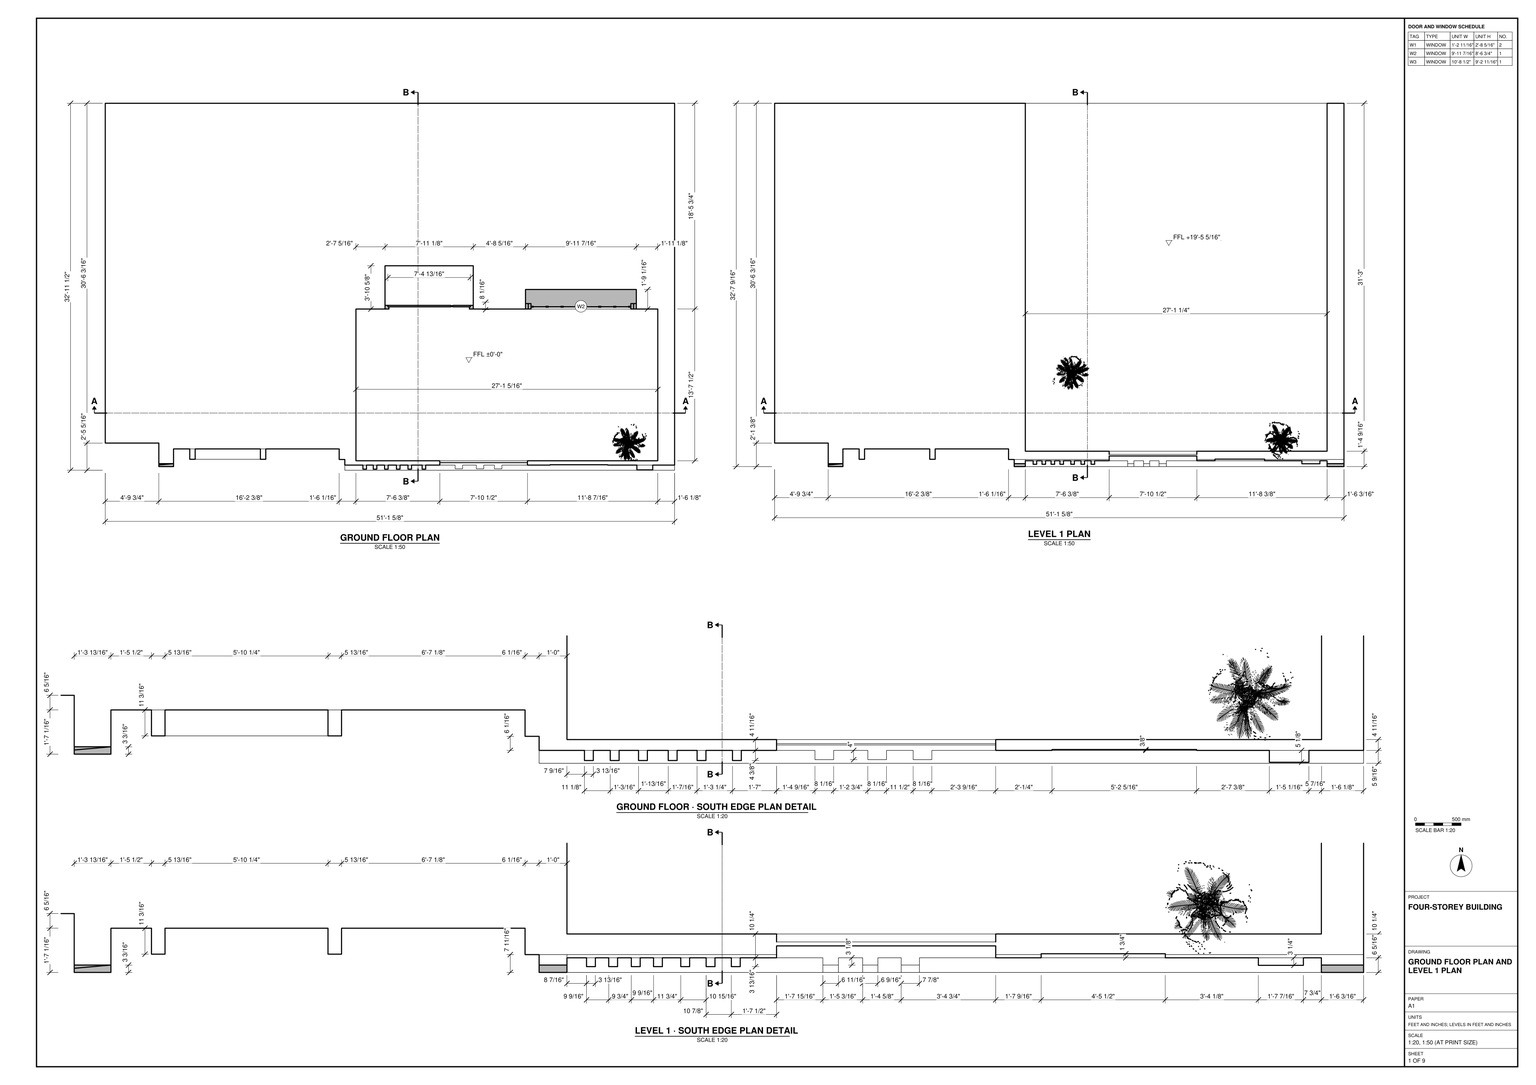
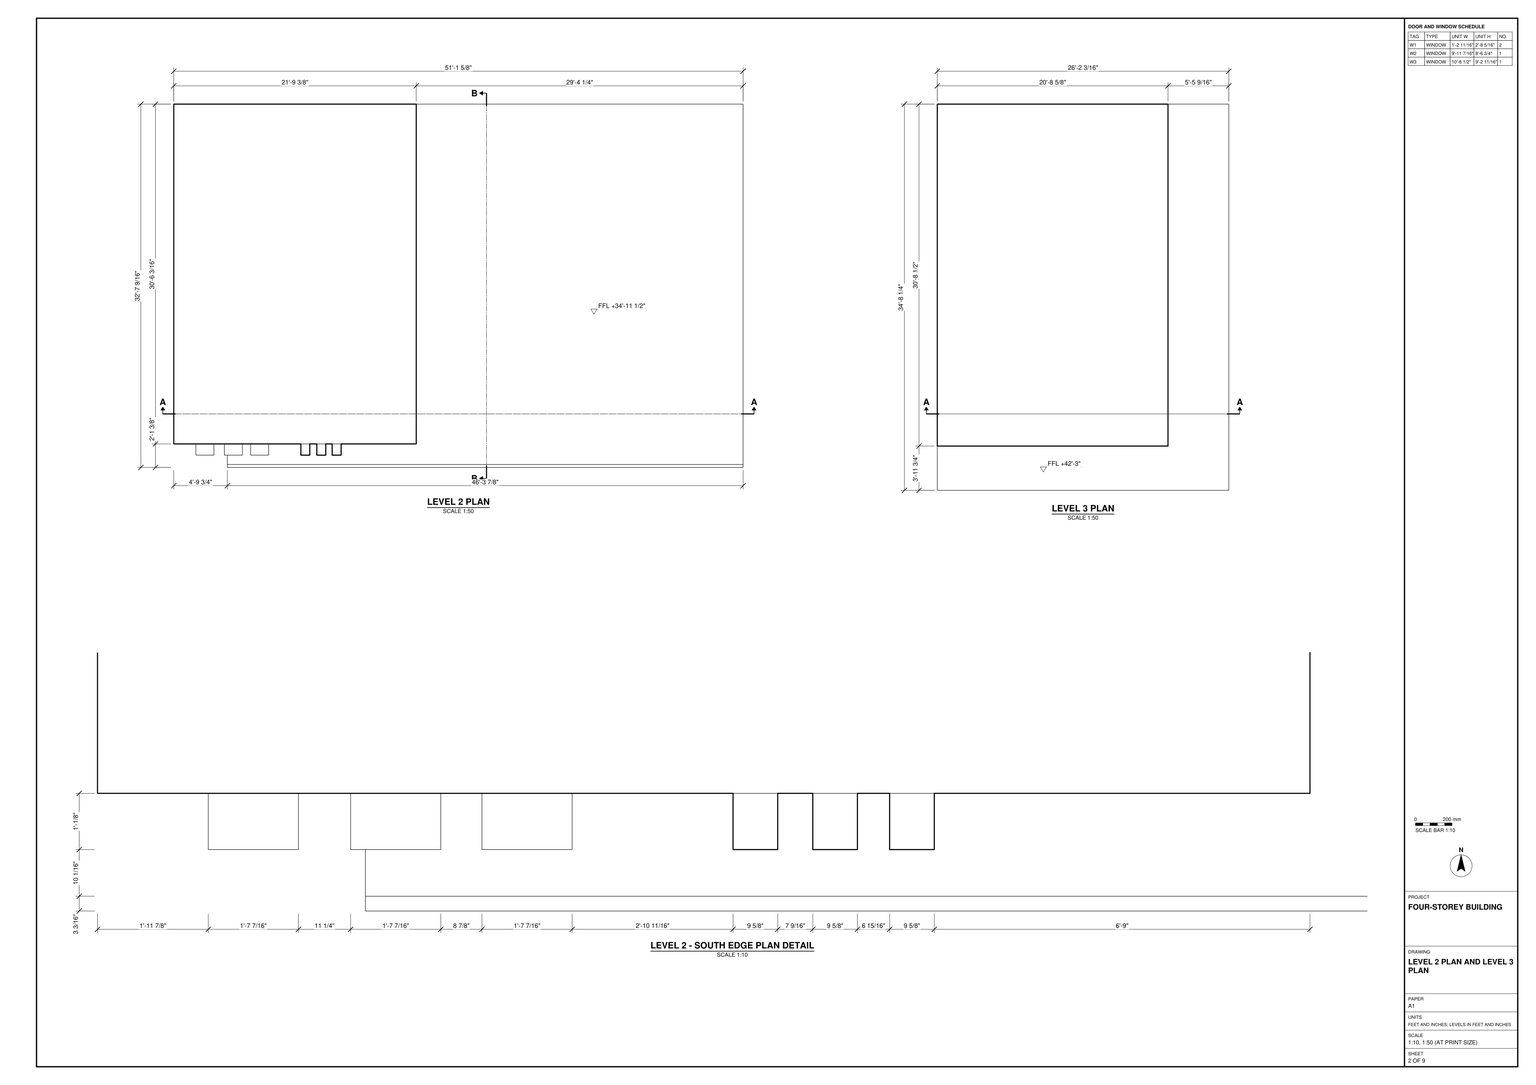
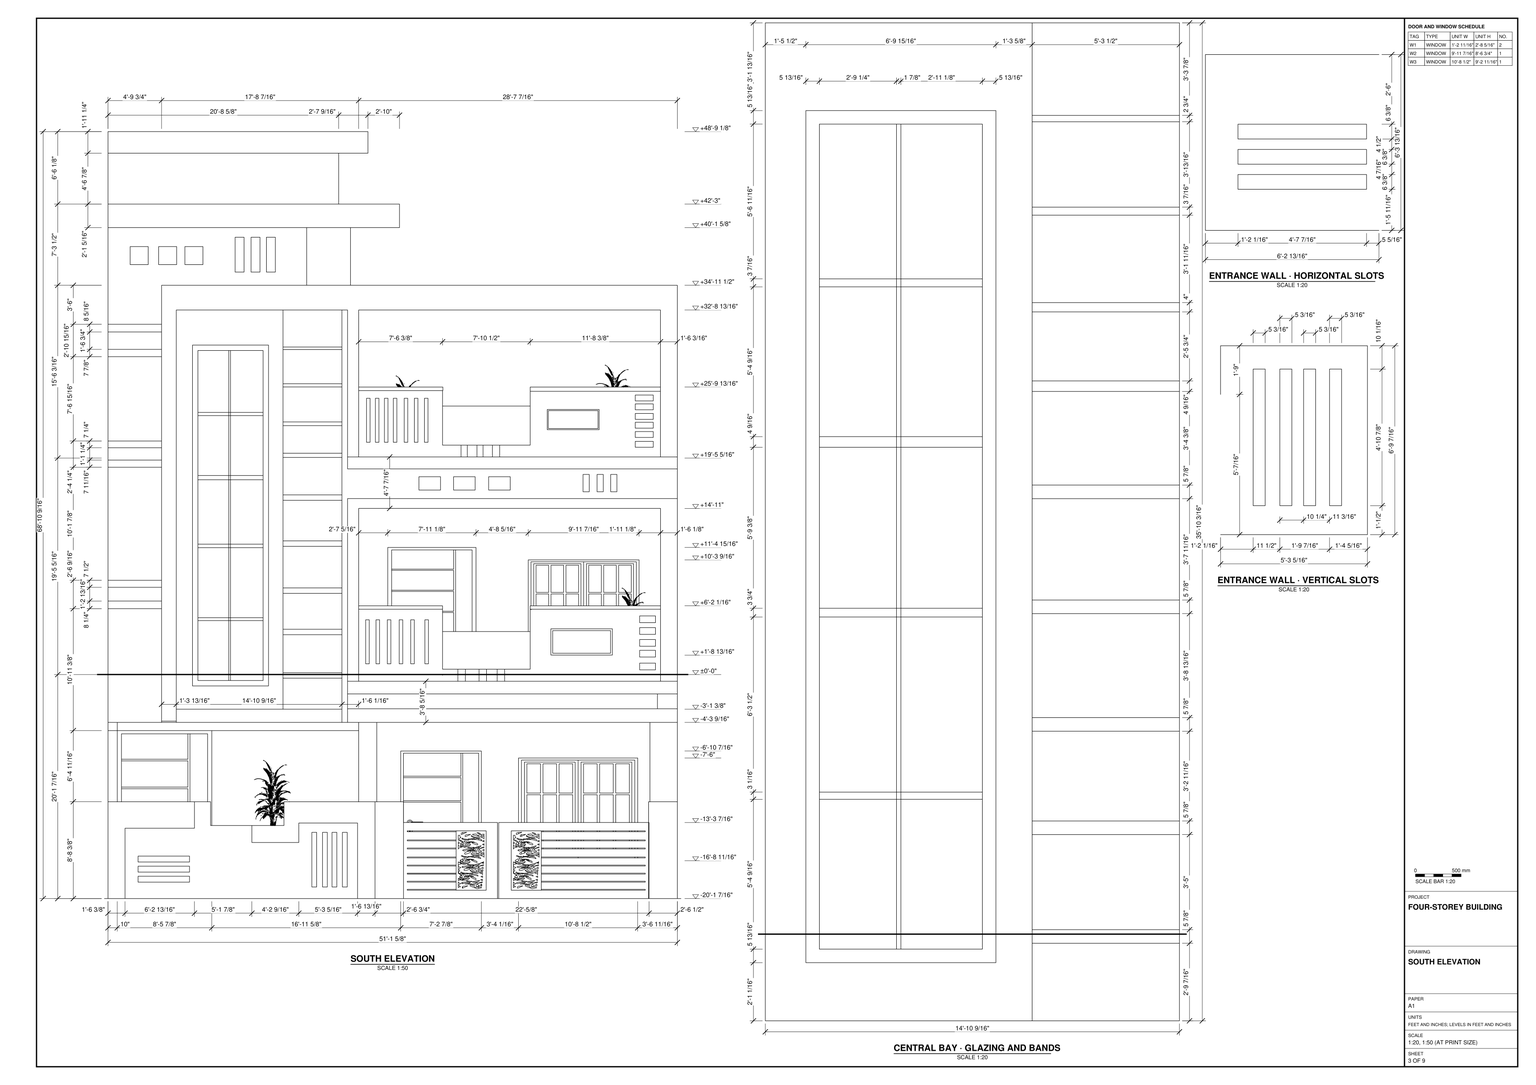
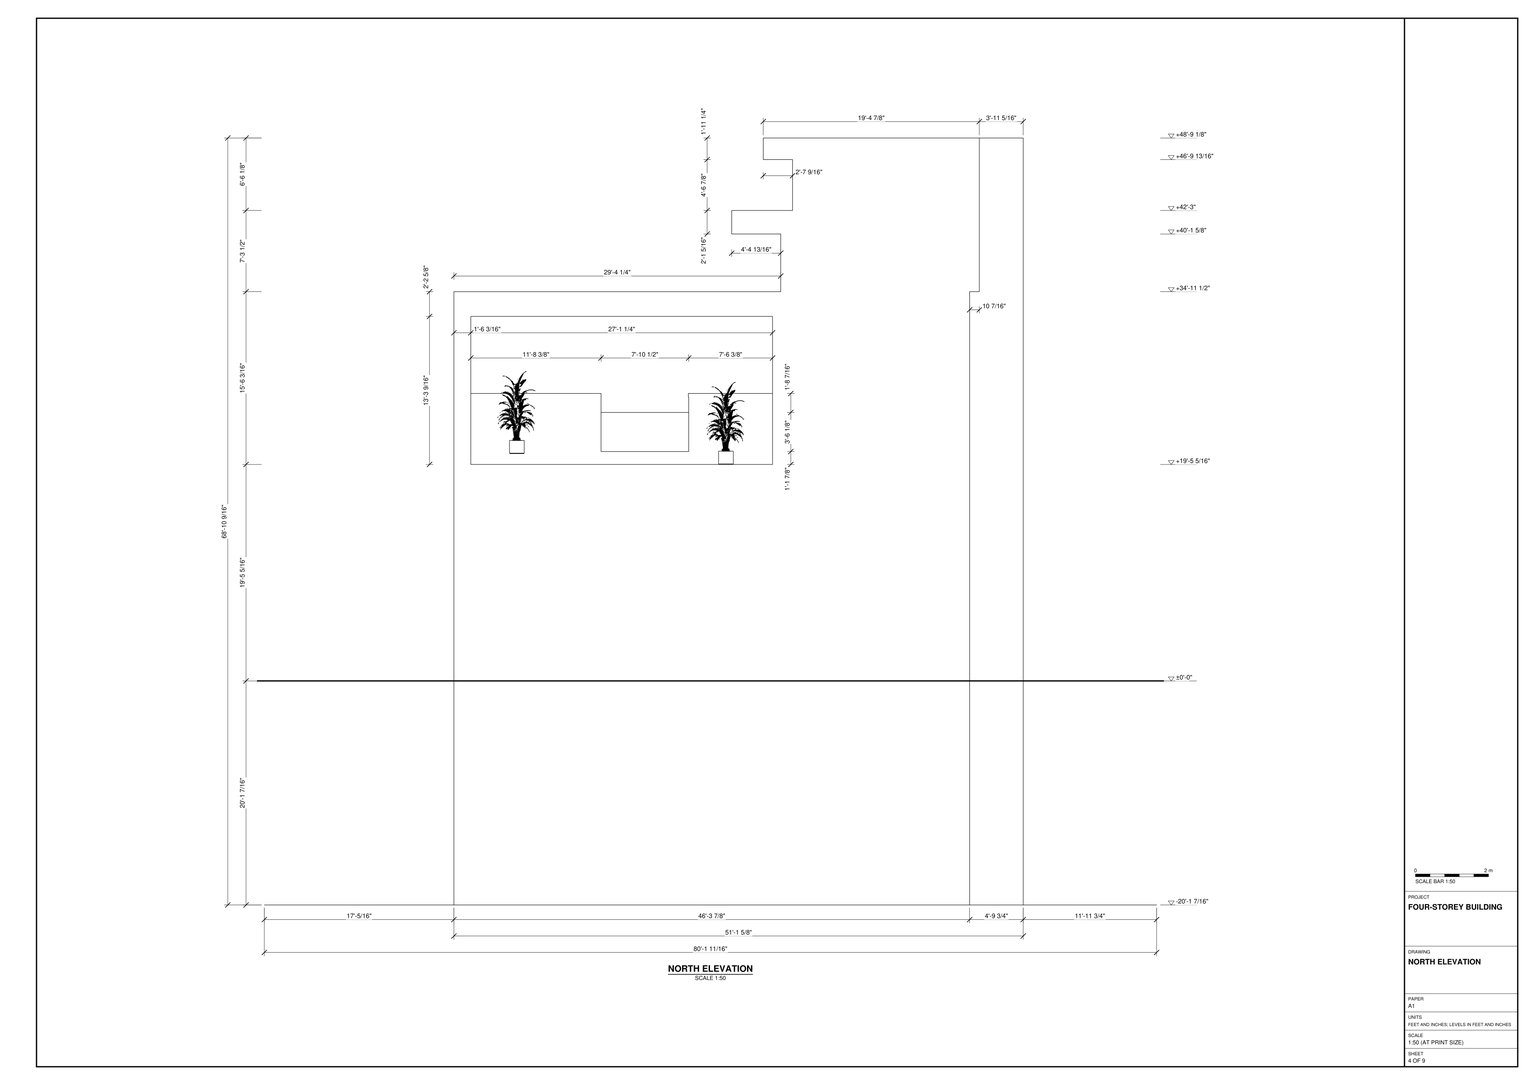
Build the four-storey building in SketchUp from task_files/diagram_01.pdf. Work in feet and inches. The complete model shall measure 80'-1 11/16" along X, 87'-11 5/8" along Y and 68'-10 9/16" along Z. Set the ground-floor datum at ±0'-0" and the successive floor levels at +19'-5 5/16", +34'-11 1/2" and +42'-3". Use the south elevation to locate the entrance frontage below the ground-floor datum.

Follow the footprint at each level rather than extruding one plan through the full height. Model the walls at their drawn thicknesses, and use the enlarged south-edge plans to shape the recesses and projections. Include the floor slabs, door and window openings, stacked balconies and the narrower upper volume with its projecting flat roof edges. On the south face, distinguish the tall divided glazing from the horizontally banded strip beside it. Reproduce the balcony parapet openings, the slotted entrance wall and the slatted gates with screen inserts. Decor and loose items, including the plants, may be any suitable library components placed where shown.

Keep walls, slabs and roof elements in separate groups or components, and do the same for each furniture or joinery piece shown. Use components for repeated parts. Save one SketchUp model as output_files/four_storey_building_and_its_south_entrance_frontage.skp.

# SketchUp Ruby script. Lengths in inches.
U = 1.inch
M = Sketchup.active_model
def pt(a) = Geom::Point3d.new(a.map { |v| v * U })
def face(e, loops, mat)
  f = e.add_face(loops[0].map { |a| pt(a) })
  loops[1..].each { |l| e.add_face(l.map { |a| pt(a) }).erase! }
  f.material = f.back_material = mat if mat
  f
end
# faces: each face lists its corners as indices into pts; further lists are holes
def faces(e, pts, list, mat = nil) = list.each { |f| face(e, (f[0].is_a?(Array) ? f : [f]).map { |l| l.map { |i| pts[i] } }, mat) }
# xy, xz, yz: faces in a plane at the given z, y or x. An outline is a flat list of corners, or four numbers for a rectangle; further outlines are holes
def ring(l) = l.size == 4 ? [[l[0], l[1]], [l[2], l[1]], [l[2], l[3]], [l[0], l[3]]] : l.each_slice(2).to_a
def flat(e, list, mat, &to3) = list.each { |f| face(e, (f[0].is_a?(Array) ? f : [f]).map { |l| ring(l).map { |u, v| to3.(u, v) } }, mat) }
def xy(e, z, list, mat = nil) = flat(e, list, mat) { |x, y| [x, y, z] }
def xz(e, y, list, mat = nil) = flat(e, list, mat) { |x, z| [x, y, z] }
def yz(e, x, list, mat = nil) = flat(e, list, mat) { |y, z| [x, y, z] }
def lines(e, pts, list) = list.each { |a, b| e.add_line(pt(pts[a]), pt(pts[b])) }
# prism: a flat outline (further loops are holes) pulled along v
def prism(e, loops, v, mat = nil)
  f = face(e, loops, mat); d = Geom::Vector3d.new(v.map { |x| x * U })
  f.pushpull(f.normal.samedirection?(d) ? d.length : -d.length)
end
def box(e, o, s, mat = nil) = prism(e, [[o, [o[0] + s[0], o[1], o[2]], [o[0] + s[0], o[1] + s[1], o[2]], [o[0], o[1] + s[1], o[2]]]], [0, 0, s[2]], mat)
def at(x, y, z, deg = 0) = Geom::Transformation.translation(pt([x, y, z])) * Geom::Transformation.rotation(ORIGIN, Z_AXIS, deg.degrees)
def axes(o, x, y, z) = Geom::Transformation.new([*x, 0, *y, 0, *z, 0, *pt(o).to_a, 1])
def part(name) = M.definitions.add(name)
# library, detail: a bought-in or finely detailed component or shape, given as its bounding box
def library(name, o, s) = part(name).tap { |d| box(d.entities, o, s) }
def detail(e, o, s) = box(e.add_group.entities, o, s)
def put(e, d, t, mat = nil) = e.add_instance(d, t).tap { |i| i.material = mat if mat }
def group(e, t, mat = nil) = e.add_group.tap { |g| g.transformation = t; g.material = mat if mat }.entities
root = M.entities
M.materials.add("Niraj_Hair_Dark").color = [109, 109, 109]
M.materials.add("[0010_Snow]").color = [255, 250, 250]
M.materials.add("[0011_Seashell]").color = [255, 245, 238]
M.materials.add("[Asphalt New]").color = [67, 60, 62]
M.materials.add("[Fencing Metal Straight]").color = [194, 195, 196]
M.materials.add("[Formica Speckled Grey]").color = [94, 105, 111]
M.materials.add("[Grass Dark Green]").color = [106, 157, 55]
M.materials.add("[Polished Concrete New]").color = [200, 200, 203]
M.materials.add("[Terrazzo Tile Accent]").color = [224, 221, 217]
M.materials.add("[Translucent Glass Gray]").color = [128, 128, 128]
M.materials["[Translucent Glass Gray]"].alpha = 0.5
M.materials.add("[Wood Board Cork]").color = [215, 201, 115]
M.materials.add("[Wood Cherry Original]").color = [152, 86, 42]
M.materials.add("[Wood Veneer 01]").color = [120, 70, 37]
c1 = part("Group2\#1")
p = [[46.8125,1.1875,0],[1.1875,1.1875,0],[1.1875,58.8125,0],[46.8125,58.8125,0]]
lines(c1.entities,p,[[0,1],[1,2],[2,3],[3,0]])
c2 = part("Group1\#1")
prism(c2.entities,[[[48,0,0],[0,0,0],[0,60,0],[48,60,0]],[[1.1875,58.8125,0],[1.1875,1.1875,0],[46.8125,1.1875,0],[46.8125,58.8125,0]]],[0,0,5.875])
put(c2.entities,c1,at(0,0,0))
c3 = part("Group4\#1")
p = [[-21.625,-1.1875,0],[-1.1875,-1.1875,0],[-1.1875,-56.4375,0],[-21.625,-56.4375,0]]
lines(c3.entities,p,[[0,1],[1,2],[2,3],[3,0]])
c4 = part("Group3\#1")
prism(c4.entities,[[[-22.8125,0,0],[0,0,0],[0,-57.625,0],[-22.8125,-57.625,0]],[[-21.625,-56.4375,0],[-1.1875,-56.4375,0],[-1.1875,-1.1875,0],[-21.625,-1.1875,0]]],[0,0,5.875])
put(c4.entities,c3,at(0,0,0))
c5 = part("Group7\#1")
p = [[21.625,1.1875,0],[1.1875,1.1875,0],[1.1875,56.4375,0],[21.625,56.4375,0]]
lines(c5.entities,p,[[0,1],[1,2],[2,3],[3,0]])
c6 = part("Group6\#1")
prism(c6.entities,[[[22.8125,0,0],[0,0,0],[0,57.625,0],[22.8125,57.625,0]],[[21.625,1.1875,0],[21.625,56.4375,0],[1.1875,56.4375,0],[1.1875,1.1875,0]]],[0,0,5.875])
put(c6.entities,c5,at(0,0,0))
c7 = part("Group10\#2")
xy(c7.entities,0,[[-9.22,-26.625,-3.74,-9.54],[-2.74,-26.625,2.74,-9.54],[3.74,-26.625,9.22,-9.54],[-9.22,-8.54,-3.74,8.54],[-2.74,-8.54,2.74,8.54],
  [3.74,-8.54,9.22,8.54],[-9.22,9.54,-3.74,26.625],[-2.74,9.54,2.74,26.625],[3.74,9.54,9.22,26.625]])
c8 = part("Group9\#1")
prism(c8.entities,[[[10.22,27.625,0],[10.22,-27.625,0],[-10.22,-27.625,0],[-10.22,27.625,0]],[[2.74,-8.54,0],[2.74,8.54,0],[-2.74,8.54,0],[-2.74,-8.54,0]],[[-2.74,-26.625,0],[2.74,-26.625,0],[2.74,-9.54,0],[-2.74,-9.54,0]],[[3.74,-9.54,0],[3.74,-26.625,0],[9.22,-26.625,0],[9.22,-9.54,0]],[[-2.74,9.54,0],[2.74,9.54,0],[2.74,26.625,0],[-2.74,26.625,0]],[[9.22,8.54,0],[3.74,8.54,0],[3.74,-8.54,0],[9.22,-8.54,0]],[[-9.22,-8.54,0],[-3.74,-8.54,0],[-3.74,8.54,0],[-9.22,8.54,0]],[[3.74,9.54,0],[9.22,9.54,0],[9.22,26.625,0],[3.74,26.625,0]],[[-3.74,26.625,0],[-9.22,26.625,0],[-9.22,9.54,0],[-3.74,9.54,0]],[[-9.22,-26.625,0],[-3.74,-26.625,0],[-3.74,-9.54,0],[-9.22,-9.54,0]]],[0,0,1])
put(c8.entities,c7,at(0,0,0.5),"[Translucent Glass Gray]")
c9 = part("Group8\#2")
xy(c9.entities,0,[[-9.22,-26.625,-3.74,-9.54],[-2.74,-26.625,2.74,-9.54],[3.74,-26.625,9.22,-9.54],[-9.22,-8.54,-3.74,8.54],[-2.74,-8.54,2.74,8.54],
  [3.74,-8.54,9.22,8.54],[-9.22,9.54,-3.74,26.625],[-2.74,9.54,2.74,26.625],[3.74,9.54,9.22,26.625]])
c10 = part("Group7\#2")
prism(c10.entities,[[[10.22,27.625,0],[10.22,-27.625,0],[-10.22,-27.625,0],[-10.22,27.625,0]],[[-9.22,-8.54,0],[-3.74,-8.54,0],[-3.74,8.54,0],[-9.22,8.54,0]],[[9.22,8.54,0],[3.74,8.54,0],[3.74,-8.54,0],[9.22,-8.54,0]],[[-2.74,-8.54,0],[2.74,-8.54,0],[2.74,8.54,0],[-2.74,8.54,0]],[[9.22,-26.625,0],[9.22,-9.54,0],[3.74,-9.54,0],[3.74,-26.625,0]],[[2.74,-9.54,0],[-2.74,-9.54,0],[-2.74,-26.625,0],[2.74,-26.625,0]],[[9.22,9.54,0],[9.22,26.625,0],[3.74,26.625,0],[3.74,9.54,0]],[[-9.22,26.625,0],[-9.22,9.54,0],[-3.74,9.54,0],[-3.74,26.625,0]],[[-2.74,26.625,0],[-2.74,9.54,0],[2.74,9.54,0],[2.74,26.625,0]],[[-3.74,-9.54,0],[-9.22,-9.54,0],[-9.22,-26.625,0],[-3.74,-26.625,0]]],[0,0,1])
put(c10.entities,c9,at(0,0,0.5),"[Translucent Glass Gray]")
c11 = part("window (1)")
g1 = group(c11.entities,at(0,140.43,0))
p = [[24,5.875,1.1875],[24,5.875,58.8125],[1.1875,5.875,1.1875],[1.1875,5.875,58.8125],[46.8125,5.875,58.8125],[46.8125,5.875,1.1875],
  [2.375,2.9375,2.375],[2.375,2.9375,57.625],[25.1875,2.9375,2.375],[25.1875,2.9375,57.625],[22.8125,2.9375,2.375],[45.625,2.9375,2.375],
  [22.8125,2.9375,57.625],[45.625,2.9375,57.625]]
lines(g1,p,[[0,1],[2,3],[4,5],[1,4],[0,2],[3,1],[5,0],[6,7],[8,9],[10,6],[11,8],[12,10],
  [7,12],[9,13],[13,11]])
put(g1,c2,axes([48,0,0],[-1,0,0],[0,0,1],[0,1,0]))
put(g1,c4,axes([1.1875,0,58.8125],[-1,0,0],[0,0,1],[0,1,0]),"[Wood Cherry Original]")
put(g1,c6,axes([46.8125,0,1.1875],[-1,0,0],[0,0,1],[0,1,0]),"[Wood Cherry Original]")
put(g1,c8,axes([35.41,1.9375,30],[-1,0,0],[0,0,1],[0,1,0]))
put(g1,c10,axes([12.59,1.9375,30],[-1,0,0],[0,0,1],[0,1,0]))
c12 = library("PINTU+6+YA",[0,-0.6875,0],[35.83,8.07,80.71])
c13 = library("NAKSHA MART",[29.67,0,0],[2606.07,274.75,1])
c14 = library("plant_176_fbx.FBX\#1",[-22.43,-22.29,0],[44.86,44.58,89.56])
c15 = part("plant")
put(c15.entities,c14,at(781.96,-582.67,447.5))
put(c15.entities,c14,at(1007.32,-654.31,459.14))
put(c15.entities,c14,at(638.98,-763.875,33.17))
put(c15.entities,c14,at(1025.54,-659,218.83))
c16 = library("Entrance canopy",[0,0,0],[98,82,12.7])
xy(root,-27.25,[[143.75,550.94,162.11,555.69],[431.51,550.94,431.51,555.69,412.72,555.69,412.72,560.82,162.11,560.82,162.11,555.69,143.75,555.69,143.75,580.65,462.25,580.65,462.25,550.94],[462.25,550.94,726.4,580.65],[727.83,716.63,727.83,736.13,546.14,736.13,546.14,769.82,459.26,769.82,459.26,736.13,433.43,736.13,433.43,718.19,413.93,718.19,413.93,730.63,255.625,730.63,255.625,769.19,201.5,769.19,201.5,1055.625,757.37,1055.625,757.37,716.63],[143.75,718.19,143.75,1055.625,201.5,1055.625,201.5,769.19,153.74,769.19,153.74,718.19]])
xy(root,-27.25,[[0,0,0,1055.625,143.75,1055.625,143.75,444.67,757.37,444.67,757.37,1055.625,961.6875,1055.625,961.6875,0]],"[Grass Dark Green]")
xy(root,-27.25,[[143.75,444.67,143.75,521.88,430.375,521.88,430.375,550.94,757.37,550.94,757.37,444.67],[143.75,521.88,430.375,550.94],[162.11,550.94,431.51,555.69],[162.11,555.69,412.72,560.82]],"[Polished Concrete New]")
xy(root,-27.25,[[143.75,580.65,143.75,718.19,153.74,718.19,153.74,769.19,255.625,769.19,255.625,730.63,413.93,730.63,413.93,718.19,433.43,718.19,433.43,736.13,459.26,736.13,459.26,769.82,546.14,769.82,546.14,736.13,727.83,736.13,727.83,716.63,757.37,716.63,757.37,580.65]],"[Terrazzo Tile Accent]")
xy(root,-14.75,[[363.45,556.19,368.63,560.82],[374.95,556.19,380.13,560.82],[385.2,556.19,390.38,560.82],[396.38,556.19,401.57,560.82]],"[Formica Speckled Grey]")
xy(root,-9.54,[[176.15,556.32,231.59,560.82]],"[Formica Speckled Grey]")
xy(root,-3.16,[[176.15,556.32,231.59,560.82]],"[Wood Veneer 01]")
xy(root,1.28,[[176.15,556.32,231.59,560.82]],"[Formica Speckled Grey]")
xy(root,7.65,[[176.15,556.32,231.59,560.82]],"[Wood Veneer 01]")
xy(root,12.15,[[176.15,556.32,231.59,560.82]],"[Formica Speckled Grey]")
xy(root,13.54,[[586.1875,736.13,714.6875,762.69]])
xy(root,18.53,[[176.15,556.32,231.59,560.82]],"[Wood Veneer 01]")
xy(root,33.18,[[298.83,555.69,349.39,560.82]])
xy(root,44.12,[[363.45,556.19,368.63,560.82],[374.95,556.19,380.13,560.82],[385.2,556.19,390.38,560.82],[396.38,556.19,401.57,560.82]],"[Formica Speckled Grey]")
xy(root,48.55,[[162.11,550.94,236.92,560.82]])
xy(root,51.49,[[298.83,555.69,333.41,560.82],[254.3,560.82,333.41,580.65]])
xy(root,54.18,[[349.39,555.69,412.72,560.82]])
xy(root,77.12,[[143.75,550.94,143.75,580.65,254.3,580.65,254.3,560.82,236.92,560.82,236.92,550.94],[726.4,550.94,757.37,580.65],[333.41,555.69,431.51,580.65]],"[0010_Snow]")
xy(root,77.12,[[431.51,550.94,462.25,580.65]],"[0011_Seashell]")
xy(root,124.23,[[586.1875,736.13,714.6875,762.69]])
xy(root,131.75,[[459.26,736.13,546.14,769.82]])
xy(root,153.79,[[153.74,718.19,413.93,718.19,413.93,730.63,255.625,730.63,255.625,769.19,153.74,769.19]])
xy(root,162.625,[[401.93,660.13,401.93,671.75,217.33,671.75,217.33,718.19,433.43,718.19,433.43,736.13,727.83,736.13,727.83,660.13],[727.83,660.13,757.37,716.63],[201.5,665.86,201.5,667.25,217.33,667.25],[201.5,667.25,217.33,718.19],[143.75,689.4375,201.5,718.19]])
xy(root,163.99,[[201.5,664.07,201.5,665.86,217.33,667.25,217.33,664.07]])
xy(root,176.85,[[217.33,671.75,395.87,683.13]])
xy(root,177.3,[[401.93,660.13,735.93,662.94],[735.93,660.13,757.37,736.13]])
xy(root,193.3,[[401.93,660.13,735.93,662.94],[735.93,660.13,757.37,736.13]])
xy(root,201.92,[[234.8125,671.94,316.75,683.13]])
xy(root,206.9375,[[401.93,660.13,757.37,660.13,757.37,665.69,571.25,665.69,571.25,661.69,563.19,661.69,563.19,665.69,551.71,665.69,551.71,661.69,543.66,661.69,543.66,665.69,528.91,665.69,528.91,661.69,520.86,661.69,520.86,665.69,401.93,665.69]])
xy(root,207.76,[[240.65,671.94,310.91,683.13]])
xy(root,214.22,[[413.93,670.36,739.25,670.36,739.25,833.88,540.38,833.88,540.38,880.5,445.26,880.5,445.26,833.88,413.93,833.88]])
xy(root,219.24,[[716.75,660.57,733.82,665.69]])
xy(root,219.97,[[520.86,661.69,528.91,661.69,528.91,665.69,543.66,665.69,543.66,661.69,551.71,661.69,551.71,665.69,563.19,665.69,563.19,661.69,571.25,661.69,571.25,665.69,598.78,665.69,598.78,668.02,504.31,668.02,504.31,665.69,520.86,665.69],[504.31,668.61,598.78,670.36]])
xy(root,225.77,[[421.48,661.32,425.29,665.69],[432.6,661.32,436.42,665.69],[444.79,661.32,448.6,665.69],[457.6,661.32,461.42,665.69],[470.04,661.32,473.85,665.69],
  [485.29,661.32,489.1,665.69]])
xy(root,226.49,[[716.75,660.57,733.82,665.69]])
xy(root,233.05,[[716.75,660.57,733.82,665.69]])
xy(root,235.01,[[596.7,833.88,716.14,854.94]],"[0010_Snow]")
xy(root,237.15,[[623.06,665.69,685.38,666.07]])
xy(root,240.3,[[716.75,660.57,733.82,665.69]])
xy(root,244.68,[[716.75,660.57,733.82,665.69]])
xy(root,251.93,[[716.75,660.57,733.82,665.69]])
xy(root,257.49,[[716.75,660.57,733.82,665.69]])
xy(root,260.53,[[504.31,668.02,598.78,668.61]])
xy(root,261.53,[[623.06,665.69,685.38,666.07]])
xy(root,264.74,[[716.75,660.57,733.82,665.69]])
xy(root,270.12,[[716.75,660.57,733.82,665.69]])
xy(root,273.21,[[421.48,661.32,425.29,665.69],[432.6,661.32,436.42,665.69],[444.79,661.32,448.6,665.69],[457.6,661.32,461.42,665.69],[470.04,661.32,473.85,665.69],
  [485.29,661.32,489.1,665.69]])
xy(root,277.37,[[716.75,660.57,733.82,665.69]])
xy(root,284.58,[[413.93,663.94,504.31,665.69],[598.78,663.94,739.25,665.69]])
xy(root,288.25,[[413.93,663.94,504.31,670.36],[598.78,663.94,739.25,670.36]])
xy(root,337.76,[[596.7,833.88,716.14,854.94]],"[0010_Snow]")
xy(root,351.15,[[445.26,833.88,540.38,880.5]],"[0010_Snow]")
xy(root,393.23,[[413.93,665.69,739.25,833.88]],"Niraj_Hair_Dark")
xy(root,403.85,[[401.93,665.69,413.93,671.75],[413.93,665.69,757.37,671.75]])
xy(root,411.17,[[655.75,666.5,662.4375,671.75],[670.875,666.5,677.5625,671.75],[685.5625,666.5,692.25,671.75]],"[0010_Snow]")
xy(root,413.01,[[478.88,657.25,502.14,671.75],[516.19,657.25,539.45,671.75],[554,657.25,577.26,671.75]],"[0010_Snow]")
xy(root,427.38,[[478.88,657.25,502.14,671.75],[516.19,657.25,539.45,671.75],[554,657.25,577.26,671.75]],"Niraj_Hair_Dark")
xy(root,429.86,[[655.75,666.5,662.4375,671.75],[670.875,666.5,677.5625,671.75],[685.5625,666.5,692.25,671.75]],"[0010_Snow]")
xy(root,435.81,[[401.93,664.07,413.93,671.75],[413.93,664.07,757.37,671.75]])
xy(root,447.5,[[413.93,680.65,739.18,1055.625]])
xy(root,448.69,[[413.93,664.07,524.26,670.38],[524.26,664.07,530.97,667.25],[530.97,664.07,541.42,670.38],[541.42,664.07,547.98,667.25],[547.98,664.07,558.04,670.38],
  [558.04,664.07,565.9,667.25],[565.9,664.07,739.18,670.38]])
xy(root,459.15,[[712.01,667.13,731.43,670.38]])
xy(root,461.41,[[524.26,667.25,530.97,667.25,530.97,670.38,541.42,670.38,541.42,667.25,547.98,667.25,547.98,670.38,558.04,670.38,558.04,667.25,565.9,667.25,565.9,670.38,598.78,670.38,598.78,675.52,504.31,675.52,504.31,670.38,524.26,670.38],[504.31,677.22,598.78,680.65]])
xy(root,464.49,[[422.375,666.57,426.1875,670.38],[431.9375,666.57,435.75,670.38],[441.6875,666.57,445.5,670.38],[451.25,666.57,455.0625,670.38],[463,666.57,466.8125,670.38],
  [473.9375,666.57,477.75,670.38],[484.8125,666.57,488.625,670.38]])
xy(root,465.49,[[712.01,667.13,731.43,670.38]])
xy(root,469.71,[[712.01,667.13,731.43,670.38]])
xy(root,476.05,[[712.01,667.13,731.43,670.38]])
xy(root,479.3,[[618.36,670.38,671.89,672.13]])
xy(root,479.71,[[712.01,667.13,731.43,670.38]])
xy(root,486.05,[[712.01,667.13,731.43,670.38]])
xy(root,489.21,[[712.01,667.13,731.43,670.38]])
xy(root,495.55,[[712.01,667.13,731.43,670.38]])
xy(root,498.63,[[618.36,670.38,671.89,672.13]])
xy(root,499.52,[[712.01,667.13,731.43,670.38]])
xy(root,505.86,[[712.01,667.13,731.43,670.38]])
xy(root,509.08,[[712.01,667.13,731.43,670.38]])
xy(root,511.93,[[422.375,666.57,426.1875,670.38],[431.9375,666.57,435.75,670.38],[441.6875,666.57,445.5,670.38],[451.25,666.57,455.0625,670.38],[463,666.57,466.8125,670.38],
  [473.9375,666.57,477.75,670.38],[484.8125,666.57,488.625,670.38]])
xy(root,515.43,[[712.01,667.13,731.43,670.38]])
xy(root,519.42,[[598.78,666,739.18,670.38]])
xy(root,520.18,[[413.93,669.69,504.68,670.38],[504.31,670.38,504.68,675.52],[504.31,675.52,504.68,677.22],[504.31,677.22,504.68,680.65]])
xy(root,524,[[598.78,666,739.18,680.65],[413.93,669.69,504.68,680.65]])
xy(root,563.4,[[240.65,671.94,310.91,683.13]])
xy(root,569.24,[[234.8125,671.94,316.75,683.13]])
xy(root,600.49,[[201.5,665.86,201.5,667.25,217.33,667.25]])
xy(root,607.05,[[217.33,664.07,395.87,683.13],[395.87,664.07,401.93,671.75],[413.93,664.07,739.18,1055.625]])
xy(root,633.6875,[[201.5,664.07,757.37,667.25]])
xy(root,633.6875,[[201.5,667.25,757.37,667.25,757.37,1055.625,405.12,1055.625,405.12,689.4375,201.5,689.4375]],"[0010_Snow]")
xy(root,647.91,[[280.75,677.3125,290.375,689.4375],[297.9375,677.3125,307.5625,689.4375],[314.5,677.3125,324.125,689.4375]])
xy(root,655.97,[[167.63,677.3125,187.06,689.4375],[198.31,677.3125,217.75,689.4375],[226.63,677.3125,246.06,689.4375]],"[0010_Snow]")
xy(root,675.41,[[167.63,677.3125,187.06,689.4375],[198.31,677.3125,217.75,689.4375],[226.63,677.3125,246.06,689.4375]],"[0010_Snow]")
xy(root,685.47,[[280.75,677.3125,290.375,689.4375],[297.9375,677.3125,307.5625,689.4375],[314.5,677.3125,324.125,689.4375]])
xy(root,695.87,[[143.75,639.38,457.93,639.38,457.93,1055.625,405.12,1055.625,405.12,689.4375,143.75,689.4375]])
xy(root,721.1875,[[143.75,639.38,457.93,639.38,457.93,1055.625,392.39,1055.625,392.39,687.1,143.75,687.1]])
xy(root,776.05,[[143.75,639.38,143.75,687.1,392.39,687.1,392.39,1055.625,423.93,1055.625,423.93,639.38]])
xy(root,799.3125,[[143.75,639.38,423.93,1055.625]])
xz(root,550.94,[[143.75,-27.25,143.75,77.12,236.92,77.12,236.92,48.55,162.11,48.55,162.11,-27.25],[431.51,-27.25,462.25,77.12],[726.4,-27.25,757.37,77.12]],"[0011_Seashell]")
xz(root,555.69,[[412.72,-27.25,412.72,54.18,349.39,54.18,349.39,33.18,298.83,33.18,298.83,51.49,333.41,51.49,333.41,77.12,431.51,77.12,431.51,-27.25]],"[0011_Seashell]")
xz(root,556.19,[[363.45,-14.75,368.63,44.12],[374.95,-14.75,380.13,44.12],[385.2,-14.75,390.38,44.12],[396.38,-14.75,401.57,44.12]],"[Wood Veneer 01]")
xz(root,556.32,[[176.15,-9.54,231.59,-3.16],[176.15,1.28,231.59,7.65],[176.15,12.15,231.59,18.53]],"[Wood Veneer 01]")
xz(root,560.82,[[[162.11,-27.25,162.11,48.55,236.92,48.55,236.92,77.12,254.3,77.12,254.3,51.49,298.83,51.49,298.83,33.18,349.39,33.18,349.39,54.18,412.72,54.18,412.72,-27.25],[176.15,12.15,231.59,18.53],[176.15,1.28,231.59,7.65],[176.15,-9.54,231.59,-3.16],[396.38,-14.75,401.57,44.12],[385.2,-14.75,390.38,44.12],[374.95,-14.75,380.13,44.12],[363.45,-14.75,368.63,44.12]]],"[Formica Speckled Grey]")
xz(root,580.65,[[143.75,-27.25,162.11,77.12],[162.11,-27.25,431.51,-27.25,431.51,77.12,333.41,77.12,333.41,51.49,254.3,51.49,254.3,77.12,162.11,77.12],[431.51,-27.25,462.25,77.12],[726.4,-27.25,757.37,77.12]])
xz(root,639.38,[[143.75,695.87,457.93,721.1875],[143.75,776.05,423.93,799.3125]],"[0011_Seashell]")
xz(root,657.25,[[478.88,413.01,502.14,427.38],[516.19,413.01,539.45,427.38],[554,413.01,577.26,427.38]],"Niraj_Hair_Dark")
xz(root,660.13,[[401.93,162.625,757.37,177.3],[401.93,193.3,757.37,206.9375]],"[0011_Seashell]")
xz(root,660.57,[[716.75,219.24,733.82,226.49],[716.75,233.05,733.82,240.3],[716.75,244.68,733.82,251.93],[716.75,257.49,733.82,264.74],[716.75,270.12,733.82,277.37]])
xz(root,661.32,[[421.48,225.77,425.29,273.21],[432.6,225.77,436.42,273.21],[444.79,225.77,448.6,273.21],[457.6,225.77,461.42,273.21],[470.04,225.77,473.85,273.21],
  [485.29,225.77,489.1,273.21]])
xz(root,661.69,[[520.86,206.9375,528.91,219.97],[543.66,206.9375,551.71,219.97],[563.19,206.9375,571.25,219.97]])
xz(root,662.94,[[401.93,177.3,735.93,193.3]])
xz(root,663.94,[[413.93,284.58,504.31,288.25],[598.78,284.58,739.25,288.25]])
xz(root,664.07,[[201.5,163.99,217.33,163.99,217.33,607.05,401.93,607.05,401.93,448.69,413.93,448.69,413.93,607.05,739.18,607.05,739.18,448.69,757.37,448.69,757.37,633.6875,201.5,633.6875],[401.93,435.81,757.37,448.69]],"[0011_Seashell]")
xz(root,665.69,[[[621.1,235.18,687.35,263.49],[623.06,237.15,685.38,261.53]]])
xz(root,665.69,[[401.93,206.9375,413.93,206.9375,413.93,393.23,739.25,393.23,739.25,206.9375,757.37,206.9375,757.37,403.85,401.93,403.85]],"[0011_Seashell]")
xz(root,665.69,[[[413.93,206.9375,520.86,206.9375,520.86,219.97,504.31,219.97,504.31,284.58,413.93,284.58],[421.48,225.77,425.29,273.21],[432.6,225.77,436.42,273.21],[444.79,225.77,448.6,273.21],[457.6,225.77,461.42,273.21],[470.04,225.77,473.85,273.21],[485.29,225.77,489.1,273.21]],[528.91,206.9375,543.66,219.97],[551.71,206.9375,563.19,219.97],[[571.25,206.9375,739.25,206.9375,739.25,284.58,598.78,284.58,598.78,219.97,571.25,219.97],[621.1,235.18,687.35,263.49],[716.75,219.24,733.82,226.49],[716.75,233.05,733.82,240.3],[716.75,244.68,733.82,251.93],[716.75,257.49,733.82,264.74],[716.75,270.12,733.82,277.37]]],"[Asphalt New]")
xz(root,666,[[598.78,519.42,739.18,524]])
xz(root,666.07,[[623.06,237.15,685.38,261.53]])
xz(root,666.5,[[655.75,411.17,662.4375,429.86],[670.875,411.17,677.5625,429.86],[685.5625,411.17,692.25,429.86]],"[0010_Snow]")
xz(root,666.57,[[422.375,464.49,426.1875,511.93],[431.9375,464.49,435.75,511.93],[441.6875,464.49,445.5,511.93],[451.25,464.49,455.0625,511.93],[463,464.49,466.8125,511.93],
  [473.9375,464.49,477.75,511.93],[484.8125,464.49,488.625,511.93]])
xz(root,667.13,[[712.01,459.15,731.43,465.49],[712.01,469.71,731.43,476.05],[712.01,479.71,731.43,486.05],[712.01,489.21,731.43,495.55],[712.01,499.52,731.43,505.86],
  [712.01,509.08,731.43,515.43]])
xz(root,667.25,[[201.5,162.625,217.33,600.49],[401.93,448.69,401.93,607.05,217.33,607.05,217.33,600.49,201.5,600.49,201.5,633.6875,757.37,633.6875,757.37,448.69,739.18,448.69,739.18,607.05,413.93,607.05,413.93,448.69],[524.26,448.69,530.97,461.41],[541.42,448.69,547.98,461.41],[558.04,448.69,565.9,461.41]])
xz(root,668.61,[[504.31,219.97,598.78,260.53]],"[Fencing Metal Straight]")
xz(root,669.69,[[413.93,520.18,504.68,524]])
xz(root,670.36,[[413.93,214.22,504.31,288.25],[504.31,214.22,598.78,219.97],[598.78,214.22,739.25,288.25]])
xz(root,670.38,[[[617.16,478.09,673.1,499.84],[618.36,479.3,671.89,498.63]]])
xz(root,670.38,[[[413.93,448.69,524.26,448.69,524.26,461.41,504.31,461.41,504.31,520.18,413.93,520.18],[484.8125,464.49,488.625,511.93],[473.9375,464.49,477.75,511.93],[463,464.49,466.8125,511.93],[451.25,464.49,455.0625,511.93],[441.6875,464.49,445.5,511.93],[431.9375,464.49,435.75,511.93],[422.375,464.49,426.1875,511.93]],[530.97,448.69,541.42,461.41],[547.98,448.69,558.04,461.41],[[565.9,448.69,739.18,448.69,739.18,519.42,598.78,519.42,598.78,461.41,565.9,461.41],[617.16,478.09,673.1,499.84],[712.01,509.08,731.43,515.43],[712.01,499.52,731.43,505.86],[712.01,489.21,731.43,495.55],[712.01,479.71,731.43,486.05],[712.01,469.71,731.43,476.05],[712.01,459.15,731.43,465.49]]],"[Asphalt New]")
xz(root,671.75,[[217.33,162.625,395.87,176.85],[[395.87,162.625,401.93,162.625,401.93,403.85,757.37,403.85,757.37,435.81,401.93,435.81,401.93,607.05,395.87,607.05],[478.88,413.01,502.14,427.38],[516.19,413.01,539.45,427.38],[554,413.01,577.26,427.38],[655.75,411.17,662.4375,429.86],[670.875,411.17,677.5625,429.86],[685.5625,411.17,692.25,429.86]]],"[0011_Seashell]")
xz(root,671.94,[[[234.8125,201.92,316.75,569.24],[240.65,207.76,310.91,563.4]]],"[0011_Seashell]")
xz(root,672.13,[[618.36,479.3,671.89,498.63]])
xz(root,675.52,[[504.31,461.41,598.78,503.55]],"[Fencing Metal Straight]")
xz(root,677.3125,[[280.75,647.91,290.375,685.47],[297.9375,647.91,307.5625,685.47],[314.5,647.91,324.125,685.47],[167.63,655.97,187.06,675.41],[198.31,655.97,217.75,675.41],
  [226.63,655.97,246.06,675.41]],"[0010_Snow]")
xz(root,680.65,[[413.93,447.5,413.93,524,504.68,524,504.68,520.18,504.31,520.18,504.31,461.41,598.78,461.41,598.78,524,739.18,524,739.18,447.5]])
xz(root,683.13,[[[217.33,176.85,332.375,607.05],[234.8125,201.92,316.75,569.24]]])
xz(root,683.13,[[273.89,207.76,275.78,272.34],[240.65,272.34,273.89,275.4375],[273.89,272.34,275.78,275.4375],[275.78,272.34,310.91,275.4375],[273.89,275.4375,275.78,350.93],
  [240.65,350.93,273.89,354.69],[273.89,350.93,275.78,354.69],[275.78,350.93,310.91,354.69],[273.89,354.69,275.78,424.09],[240.65,424.09,273.89,428.68],
  [273.89,424.09,275.78,428.68],[275.78,424.09,310.91,428.68],[273.89,428.68,275.78,493.25],[240.65,493.25,273.89,496.69],[273.89,493.25,275.78,496.69],
  [275.78,493.25,310.91,496.69],[273.89,496.69,275.78,563.4]],"[Asphalt New]")
xz(root,683.13,[[240.65,207.76,273.89,272.34],[275.78,207.76,310.91,272.34],[240.65,275.4375,273.89,350.93],[275.78,275.4375,310.91,350.93],[240.65,354.69,273.89,424.09],
  [275.78,354.69,310.91,424.09],[240.65,428.68,273.89,493.25],[275.78,428.68,310.91,493.25],[240.65,496.69,273.89,563.4],[275.78,496.69,310.91,563.4]],"[Translucent Glass Gray]")
xz(root,683.13,[[332.375,210.28,395.87,216.14],[332.375,257.13,395.87,262.99],[332.375,301.69,395.87,307.56],[332.375,352.38,395.87,358.24],[332.375,401.94,395.87,407.81],
  [332.375,448.16,395.87,452.7],[332.375,482.45,395.87,486.44],[332.375,524.15,395.87,527.6],[332.375,564.4,395.87,567.15]],"[Wood Board Cork]")
xz(root,683.13,[[332.375,176.85,395.87,210.28],[332.375,216.14,395.87,257.13],[332.375,262.99,395.87,301.69],[332.375,307.56,395.87,352.38],[332.375,358.24,395.87,401.94],
  [332.375,407.81,395.87,448.16],[332.375,452.7,395.87,482.45],[332.375,486.44,395.87,524.15],[332.375,527.6,395.87,564.4],[332.375,567.15,395.87,607.05]],"[Wood Veneer 01]")
xz(root,687.1,[[143.75,721.1875,392.39,776.05]],"[Asphalt New]")
xz(root,689.4375,[[143.75,445.31,201.5,458.58]],"Niraj_Hair_Dark")
xz(root,689.4375,[[143.75,285.1875,201.5,293.41],[143.75,308.22,201.5,315.75],[143.75,437.6,201.5,445.31],[143.75,458.58,201.5,465.84],[143.75,556.75,201.5,564.64],
  [143.75,583.38,201.5,591.66]],"[0010_Snow]")
xz(root,689.4375,[[357.9,633.6875,405.12,695.87]],"[0011_Seashell]")
xz(root,689.4375,[[143.75,162.625,201.5,285.1875],[143.75,293.41,201.5,308.22],[143.75,315.75,201.5,437.6],[143.75,465.84,201.5,556.75],[143.75,564.64,201.5,583.38],
  [[143.75,591.66,143.75,695.87,357.9,695.87,357.9,633.6875,201.5,633.6875,201.5,591.66],[167.63,655.97,187.06,675.41],[198.31,655.97,217.75,675.41],[226.63,655.97,246.06,675.41],[280.75,647.91,290.375,685.47],[297.9375,647.91,307.5625,685.47],[314.5,647.91,324.125,685.47]]],"[Asphalt New]")
xz(root,716.63,[[727.83,-27.25,757.37,162.625]],"[0011_Seashell]")
xz(root,718.19,[[143.75,153.79,153.74,162.625],[153.74,153.79,413.93,162.625]],"[0010_Snow]")
xz(root,718.19,[[143.75,-27.25,153.74,153.79],[413.93,-27.25,433.43,162.625]],"[0011_Seashell]")
xz(root,730.63,[[255.625,-27.25,413.93,153.79]],"[0011_Seashell]")
xz(root,736.13,[[735.93,177.3,757.37,193.3]])
xz(root,736.13,[[[433.43,-27.25,459.26,-27.25,459.26,131.75,546.14,131.75,546.14,-27.25,727.83,-27.25,727.83,162.625,433.43,162.625],[586.1875,13.54,714.6875,124.23]]],"[0011_Seashell]")
xz(root,762.69,[[586.1875,13.54,714.6875,124.23]])
xz(root,769.19,[[153.74,-27.25,255.625,153.79]],"[0010_Snow]")
xz(root,769.82,[[459.26,-27.25,546.14,131.75]])
xz(root,833.88,[[[413.93,214.22,445.26,214.22,445.26,351.15,540.38,351.15,540.38,214.22,739.25,214.22,739.25,393.23,413.93,393.23],[596.7,235.01,716.14,337.76]]],"[0011_Seashell]")
xz(root,854.94,[[596.7,235.01,716.14,337.76]],"[0010_Snow]")
xz(root,880.5,[[445.26,214.22,540.38,351.15]],"[0010_Snow]")
xz(root,1055.625,[[143.75,-27.25,201.5,-27.25,201.5,633.6875,191.06,633.6875,191.06,799.3125,143.75,799.3125],[[201.5,-27.25,201.5,633.6875,191.06,633.6875,191.06,799.3125,423.93,799.3125,423.93,776.05,392.39,776.05,392.39,721.1875,457.93,721.1875,457.93,695.87,405.12,695.87,405.12,633.6875,757.37,633.6875,757.37,-27.25],[413.93,447.5,739.18,607.05]]])
yz(root,143.75,[[550.94,-27.25,580.65,77.12],[718.19,-27.25,1055.625,-27.25,1055.625,799.3125,639.38,799.3125,639.38,776.05,687.1,776.05,687.1,721.1875,639.38,721.1875,639.38,695.87,689.4375,695.87,689.4375,162.625,718.19,162.625]])
yz(root,153.74,[[718.19,-27.25,769.19,153.79]])
yz(root,162.11,[[550.94,-27.25,560.82,48.55]])
yz(root,167.63,[[677.3125,655.97,689.4375,675.41]],"[0010_Snow]")
yz(root,176.15,[[556.32,-9.54,560.82,-3.16],[556.32,1.28,560.82,7.65],[556.32,12.15,560.82,18.53]],"[Formica Speckled Grey]")
yz(root,187.06,[[677.3125,655.97,689.4375,675.41]],"[0010_Snow]")
yz(root,198.31,[[677.3125,655.97,689.4375,675.41]],"[0010_Snow]")
yz(root,201.5,[[665.86,162.625,667.25,600.49],[667.25,162.625,689.4375,633.6875],[664.07,163.99,665.86,163.99,665.86,600.49,667.25,600.49,667.25,633.6875,664.07,633.6875]])
yz(root,217.33,[[667.25,162.625,671.75,162.625,671.75,176.85,683.13,176.85,683.13,607.05,667.25,607.05],[664.07,163.99,667.25,607.05]])
yz(root,217.75,[[677.3125,655.97,689.4375,675.41]],"[0010_Snow]")
yz(root,226.63,[[677.3125,655.97,689.4375,675.41]],"[0010_Snow]")
yz(root,231.59,[[556.32,-9.54,560.82,-3.16],[556.32,1.28,560.82,7.65],[556.32,12.15,560.82,18.53]],"[Formica Speckled Grey]")
yz(root,234.8125,[[671.94,201.92,683.13,569.24]])
yz(root,236.92,[[550.94,48.55,560.82,77.12]])
yz(root,240.65,[[671.94,207.76,683.13,563.4]])
yz(root,246.06,[[677.3125,655.97,689.4375,675.41]],"[0010_Snow]")
yz(root,254.3,[[560.82,51.49,580.65,77.12]])
yz(root,255.625,[[730.63,-27.25,769.19,153.79]],"[0010_Snow]")
yz(root,280.75,[[677.3125,647.91,689.4375,685.47]],"[0010_Snow]")
yz(root,290.375,[[677.3125,647.91,689.4375,685.47]],"[0010_Snow]")
yz(root,297.9375,[[677.3125,647.91,689.4375,685.47]],"[0010_Snow]")
yz(root,298.83,[[555.69,33.18,560.82,51.49]])
yz(root,307.5625,[[677.3125,647.91,689.4375,685.47]],"[0010_Snow]")
yz(root,310.91,[[671.94,207.76,683.13,563.4]])
yz(root,314.5,[[677.3125,647.91,689.4375,685.47]],"[0010_Snow]")
yz(root,316.75,[[671.94,201.92,683.13,569.24]])
yz(root,324.125,[[677.3125,647.91,689.4375,685.47]],"[0010_Snow]")
yz(root,333.41,[[555.69,51.49,560.82,77.12],[560.82,51.49,580.65,77.12]])
yz(root,349.39,[[555.69,33.18,560.82,54.18]])
yz(root,363.45,[[556.19,-14.75,560.82,44.12]],"[Wood Veneer 01]")
yz(root,368.63,[[556.19,-14.75,560.82,44.12]],"[Wood Veneer 01]")
yz(root,374.95,[[556.19,-14.75,560.82,44.12]],"[Wood Veneer 01]")
yz(root,380.13,[[556.19,-14.75,560.82,44.12]],"[Wood Veneer 01]")
yz(root,385.2,[[556.19,-14.75,560.82,44.12]],"[Wood Veneer 01]")
yz(root,390.38,[[556.19,-14.75,560.82,44.12]],"[Wood Veneer 01]")
yz(root,392.39,[[687.1,721.1875,1055.625,776.05]])
yz(root,395.87,[[671.75,176.85,683.13,607.05]])
yz(root,396.38,[[556.19,-14.75,560.82,44.12]],"[Wood Veneer 01]")
yz(root,401.57,[[556.19,-14.75,560.82,44.12]],"[Wood Veneer 01]")
yz(root,401.93,[[660.13,162.625,660.13,177.3,662.94,177.3,662.94,193.3,660.13,193.3,660.13,206.9375,671.75,206.9375,671.75,162.625],[665.69,206.9375,671.75,403.85],[664.07,435.81,671.75,607.05]])
yz(root,405.12,[[689.4375,633.6875,1055.625,695.87]])
yz(root,412.72,[[555.69,-27.25,560.82,54.18]])
yz(root,413.93,[[718.19,-27.25,730.63,0],[718.19,0,730.63,153.79],[670.36,214.22,833.88,214.22,833.88,263.625,748.25,263.625,748.25,393.23,665.69,393.23,665.69,288.25,670.36,288.25],[748.25,263.625,833.88,393.23],[663.94,284.58,665.69,288.25],
  [680.65,447.5,1055.625,447.5,1055.625,607.05,664.07,607.05,664.07,498.75,670.38,498.75,670.38,520.18,669.69,520.18,669.69,524,680.65,524],[664.07,448.69,667.25,498.75],[667.25,448.69,670.38,498.75]])
yz(root,421.48,[[661.32,225.77,665.69,273.21]])
yz(root,422.375,[[666.57,464.49,670.38,511.93]])
yz(root,423.93,[[639.38,776.05,1055.625,799.3125]])
yz(root,425.29,[[661.32,225.77,665.69,273.21]])
yz(root,426.1875,[[666.57,464.49,670.38,511.93]])
yz(root,431.51,[[550.94,-27.25,555.69,77.12]])
yz(root,431.9375,[[666.57,464.49,670.38,511.93]])
yz(root,432.6,[[661.32,225.77,665.69,273.21]])
yz(root,433.43,[[718.19,-27.25,736.13,0],[718.19,0,736.13,162.625]])
yz(root,435.75,[[666.57,464.49,670.38,511.93]])
yz(root,436.42,[[661.32,225.77,665.69,273.21]])
yz(root,441.6875,[[666.57,464.49,670.38,511.93]])
yz(root,444.79,[[661.32,225.77,665.69,273.21]])
yz(root,445.26,[[833.88,214.22,880.5,351.15]],"[0010_Snow]")
yz(root,445.5,[[666.57,464.49,670.38,511.93]])
yz(root,448.6,[[661.32,225.77,665.69,273.21]])
yz(root,451.25,[[666.57,464.49,670.38,511.93]])
yz(root,455.0625,[[666.57,464.49,670.38,511.93]])
yz(root,457.6,[[661.32,225.77,665.69,273.21]])
yz(root,457.93,[[639.38,695.87,1055.625,721.1875]],"[0010_Snow]")
yz(root,459.26,[[736.13,-27.25,769.82,131.75]])
yz(root,461.42,[[661.32,225.77,665.69,273.21]])
yz(root,462.25,[[550.94,-27.25,580.65,77.12]],"[0010_Snow]")
yz(root,463,[[666.57,464.49,670.38,511.93]])
yz(root,466.8125,[[666.57,464.49,670.38,511.93]])
yz(root,470.04,[[661.32,225.77,665.69,273.21]])
yz(root,473.85,[[661.32,225.77,665.69,273.21]])
yz(root,473.9375,[[666.57,464.49,670.38,511.93]])
yz(root,477.75,[[666.57,464.49,670.38,511.93]])
yz(root,478.88,[[657.25,413.01,671.75,427.38]],"Niraj_Hair_Dark")
yz(root,484.8125,[[666.57,464.49,670.38,511.93]])
yz(root,485.29,[[661.32,225.77,665.69,273.21]])
yz(root,488.625,[[666.57,464.49,670.38,511.93]])
yz(root,489.1,[[661.32,225.77,665.69,273.21]])
yz(root,502.14,[[657.25,413.01,671.75,427.38]],"Niraj_Hair_Dark")
yz(root,504.31,[[665.69,219.97,668.02,219.97,668.02,260.53,668.61,260.53,668.61,219.97,670.36,219.97,670.36,288.25,663.94,288.25,663.94,284.58,665.69,284.58],[670.38,461.41,675.52,520.18],[677.22,461.41,680.65,520.18]])
yz(root,504.68,[[669.69,520.18,680.65,524]])
yz(root,516.19,[[657.25,413.01,671.75,427.38]],"Niraj_Hair_Dark")
yz(root,520.86,[[661.69,206.9375,665.69,219.97]])
yz(root,524.26,[[667.25,448.69,670.38,461.41]])
yz(root,528.91,[[661.69,206.9375,665.69,219.97]])
yz(root,530.97,[[667.25,448.69,670.38,461.41]])
yz(root,539.45,[[657.25,413.01,671.75,427.38]],"Niraj_Hair_Dark")
yz(root,540.38,[[833.88,214.22,880.5,351.15]],"[0010_Snow]")
yz(root,541.42,[[667.25,448.69,670.38,461.41]])
yz(root,543.66,[[661.69,206.9375,665.69,219.97]])
yz(root,546.14,[[736.13,-27.25,769.82,131.75]])
yz(root,547.98,[[667.25,448.69,670.38,461.41]])
yz(root,551.71,[[661.69,206.9375,665.69,219.97]])
yz(root,554,[[657.25,413.01,671.75,427.38]],"Niraj_Hair_Dark")
yz(root,558.04,[[667.25,448.69,670.38,461.41]])
yz(root,563.19,[[661.69,206.9375,665.69,219.97]])
yz(root,565.9,[[667.25,448.69,670.38,461.41]])
yz(root,571.25,[[661.69,206.9375,665.69,219.97]])
yz(root,577.26,[[657.25,413.01,671.75,427.38]],"Niraj_Hair_Dark")
yz(root,586.1875,[[736.13,13.54,762.69,124.23]])
yz(root,596.7,[[833.88,235.01,854.94,337.76]],"[0010_Snow]")
yz(root,598.78,[[665.69,219.97,665.69,284.58,663.94,284.58,663.94,288.25,670.36,288.25,670.36,219.97,668.61,219.97,668.61,260.53,668.02,260.53,668.02,219.97],[670.38,461.41,670.38,519.42,666,519.42,666,524,680.65,524,680.65,461.41,677.22,461.41,677.22,520.18,675.52,520.18,675.52,461.41]])
yz(root,618.36,[[670.38,479.3,672.13,498.63]])
yz(root,623.06,[[665.69,237.15,666.07,261.53]])
yz(root,655.75,[[666.5,411.17,671.75,429.86]],"[0010_Snow]")
yz(root,662.4375,[[666.5,411.17,671.75,429.86]],"[0010_Snow]")
yz(root,670.875,[[666.5,411.17,671.75,429.86]],"[0010_Snow]")
yz(root,671.89,[[670.38,479.3,672.13,498.63]])
yz(root,677.5625,[[666.5,411.17,671.75,429.86]],"[0010_Snow]")
yz(root,685.38,[[665.69,237.15,666.07,261.53]])
yz(root,685.5625,[[666.5,411.17,671.75,429.86]],"[0010_Snow]")
yz(root,692.25,[[666.5,411.17,671.75,429.86]],"[0010_Snow]")
yz(root,712.01,[[667.13,459.15,670.38,465.49],[667.13,469.71,670.38,476.05],[667.13,479.71,670.38,486.05],[667.13,489.21,670.38,495.55],[667.13,499.52,670.38,505.86],
  [667.13,509.08,670.38,515.43]])
yz(root,714.6875,[[736.13,13.54,762.69,124.23]])
yz(root,716.14,[[833.88,235.01,854.94,337.76]],"[0010_Snow]")
yz(root,716.75,[[660.57,219.24,665.69,226.49],[660.57,233.05,665.69,240.3],[660.57,244.68,665.69,251.93],[660.57,257.49,665.69,264.74],[660.57,270.12,665.69,277.37]])
yz(root,726.4,[[550.94,-27.25,580.65,77.12]],"[0010_Snow]")
yz(root,727.83,[[716.63,-27.25,736.13,0],[716.63,0,736.13,162.625]])
yz(root,731.43,[[667.13,459.15,670.38,465.49],[667.13,469.71,670.38,476.05],[667.13,479.71,670.38,486.05],[667.13,489.21,670.38,495.55],[667.13,499.52,670.38,505.86],
  [667.13,509.08,670.38,515.43]])
yz(root,733.82,[[660.57,219.24,665.69,226.49],[660.57,233.05,665.69,240.3],[660.57,244.68,665.69,251.93],[660.57,257.49,665.69,264.74],[660.57,270.12,665.69,277.37]])
yz(root,735.93,[[662.94,177.3,736.13,193.3]])
yz(root,739.18,[[680.65,447.5,680.65,524,667.25,524,667.25,607.05,1055.625,607.05,1055.625,447.5],[664.07,448.69,667.25,498.75],[667.25,448.69,670.38,498.75],[664.07,498.75,664.07,607.05,667.25,607.05,667.25,524,666,524,666,519.42,667.25,519.42,667.25,498.75],[667.25,498.75,670.38,519.42]])
yz(root,739.25,[[670.36,214.22,670.36,288.25,665.69,288.25,665.69,393.23,833.88,393.23,833.88,214.22],[663.94,284.58,665.69,288.25]])
yz(root,757.37,[[550.94,-27.25,580.65,77.12],[716.63,-27.25,1055.625,-27.25,1055.625,407.25,748.25,407.25,748.25,180.1875,736.13,180.1875,736.13,162.625,716.63,162.625],[660.13,162.625,736.13,177.3],[736.13,180.1875,748.25,180.1875,748.25,407.25,671.75,407.25,671.75,403.85,665.69,403.85,665.69,206.9375,736.13,206.9375],[660.13,193.3,736.13,206.9375],
  [671.75,407.25,1055.625,407.25,1055.625,633.6875,664.07,633.6875,664.07,435.81,671.75,435.81]])
p = [[201.5,665.86,162.625],[217.33,667.25,162.625],[217.33,667.25,163.99],[201.5,665.86,163.99],[217.33,667.25,600.49],[201.5,665.86,600.49],
  [757.37,665.86,0],[757.37,716.63,0],[413.93,748.25,180.1875],[413.93,748.25,214.22],[413.93,683.13,180.1875],[201.5,730.63,162.625],
  [201.5,718.19,162.625],[504.31,670.38,206.9375],[504.31,665.69,214.22],[651.6,665.69,263.81],[651.6,689.88,263.81],[598.78,665.69,284.58],
  [757.37,667.25,448.69],[757.37,665.86,448.69],[401.93,667.25,448.69],[401.93,665.86,448.69]]
faces(root,p,[[0,1,2,3],[4,5,3,2]])
lines(root,p,[[6,7],[8,9],[10,8],[11,12],[13,14],[15,16],[16,17],[18,19],[20,21]])
put(root,c11,axes([586.1875,595.7,13.54],[2.67708,0,0],[0,1,0],[0,0,1.84479]))
put(root,c11,axes([596.7,693.45,235.01],[2.48828,0,0],[0,1,0],[0,0,1.7125]))
put(root,c12,axes([445.26,833.88,214.22],[2.65492,0,0],[0,1,0],[0,0,1.69669]))
put(root,c12,axes([153.74,730.63,-27.25],[2.84343,0,0],[0,1,0],[0,0,2.24311]))
put(root,c12,axes([459.26,752.09,-27.25],[2.42466,0,0],[0,-1.16159,0],[0,0,1.97005]))
put(root,c13,axes([495.23,671.94,164.11],[0.0858,0,0],[0,0,0.0858],[0,-1,0]))
put(root,c15,at(-317.73,1346.98,0))
put(root,c16,axes([726.85,550.94,-27.25],[-2.7,0,0],[0,0,1],[0,1.69,0]))
